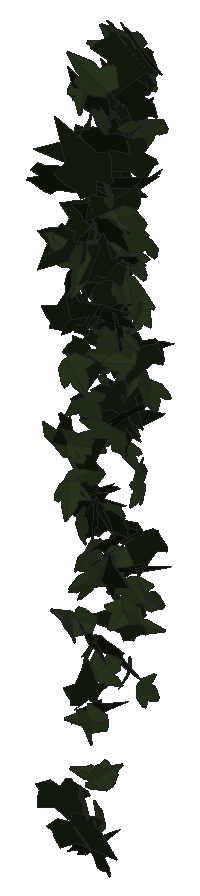
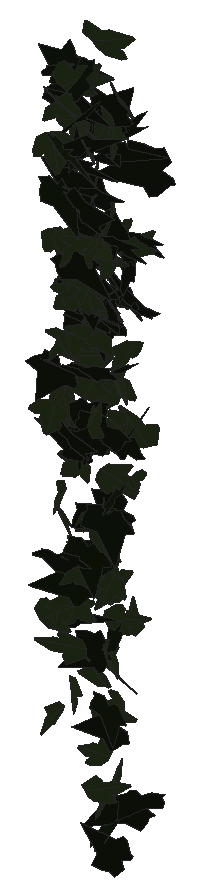
# SketchUp Ruby script. Lengths in inches.
U = 1.inch
M = Sketchup.active_model
def pt(a) = Geom::Point3d.new(a.map { |v| v * U })
def face(e, loops, mat)
  f = e.add_face(loops[0].map { |a| pt(a) })
  loops[1..].each { |l| e.add_face(l.map { |a| pt(a) }).erase! }
  f.material = f.back_material = mat if mat
  f
end
# faces: each face lists its corners as indices into pts; further lists are holes
def faces(e, pts, list, mat = nil) = list.each { |f| face(e, (f[0].is_a?(Array) ? f : [f]).map { |l| l.map { |i| pts[i] } }, mat) }
# xy, xz, yz: faces in a plane at the given z, y or x. An outline is a flat list of corners, or four numbers for a rectangle; further outlines are holes
def ring(l) = l.size == 4 ? [[l[0], l[1]], [l[2], l[1]], [l[2], l[3]], [l[0], l[3]]] : l.each_slice(2).to_a
def flat(e, list, mat, &to3) = list.each { |f| face(e, (f[0].is_a?(Array) ? f : [f]).map { |l| ring(l).map { |u, v| to3.(u, v) } }, mat) }
def xy(e, z, list, mat = nil) = flat(e, list, mat) { |x, y| [x, y, z] }
def xz(e, y, list, mat = nil) = flat(e, list, mat) { |x, z| [x, y, z] }
def yz(e, x, list, mat = nil) = flat(e, list, mat) { |y, z| [x, y, z] }
def lines(e, pts, list) = list.each { |a, b| e.add_line(pt(pts[a]), pt(pts[b])) }
# prism: a flat outline (further loops are holes) pulled along v
def prism(e, loops, v, mat = nil)
  f = face(e, loops, mat); d = Geom::Vector3d.new(v.map { |x| x * U })
  f.pushpull(f.normal.samedirection?(d) ? d.length : -d.length)
end
def box(e, o, s, mat = nil) = prism(e, [[o, [o[0] + s[0], o[1], o[2]], [o[0] + s[0], o[1] + s[1], o[2]], [o[0], o[1] + s[1], o[2]]]], [0, 0, s[2]], mat)
def at(x, y, z, deg = 0) = Geom::Transformation.translation(pt([x, y, z])) * Geom::Transformation.rotation(ORIGIN, Z_AXIS, deg.degrees)
def axes(o, x, y, z) = Geom::Transformation.new([*x, 0, *y, 0, *z, 0, *pt(o).to_a, 1])
def part(name) = M.definitions.add(name)
# library, detail: a bought-in or finely detailed component or shape, given as its bounding box
def library(name, o, s) = part(name).tap { |d| box(d.entities, o, s) }
def detail(e, o, s) = box(e.add_group.entities, o, s)
def put(e, d, t, mat = nil) = e.add_instance(d, t).tap { |i| i.material = mat if mat }
def group(e, t, mat = nil) = e.add_group.tap { |g| g.transformation = t; g.material = mat if mat }.entities
root = M.entities
M.materials.add("1026 AP 7946 SUNNY SIDE UP").color = [254, 231, 186]
M.materials.add("efeu1").color = [18, 25, 13]
M.materials.add("efeu2").color = [43, 57, 29]
c1 = part("ivyleaf_10")
p = [[0,0.5,-0.03],[-0.0625,2.02,-0.43],[-0.19,2.01,-0.46],[-0.54,1.05,-0.29],[-0.52,0.625,-0.18],[-0.83,0.76,-0.28],
  [-1.16,0.64,-0.33],[-1.15,0.33,-0.24],[-0.77,-0.39,0.02],[-0.3,-0.51,0.16],[0.04,-0.48,0.23],[-0.02,2.01,-0.4375],
  [-0.06,2.01,-0.43],[0.04,-0.49,0.23],[0.67,-0.49,0.14],[1.38,0.36,-0.2],[1.375,0.51,-0.24],[0.81,0.65,-0.19],
  [0.62,0.59,-0.15],[0.6,1.09,-0.28],[0.5,1.23,-0.31]]
faces(c1.entities,p,[[0,1,2,3,4,5,6,7,8,9,10],[11,12,0,13,14,15,16,17,18,19,20]],"efeu2")
c2 = part("ivyleaf_9")
p = [[1.54,2.16,1.25],[1.36,2.04,1.19],[-0.21,0.99,0.68],[-0.71,1.11,0.82],[-0.85,0.86,0.67],[-0.8,0.17,0.21],
  [-0.9,-0.01,0.1],[-0.67,-0.16,-0.02],[-0.08,-0.08,-0.05],[-0.03,-0.6,-0.4],[0.65,-0.88,-0.66],[0.83,-0.6,-0.49],
  [1.29,-0.42,-0.43],[1.8125,-0.07,-0.26],[1.21,0.44,0.15]]
faces(c2.entities,p,[[0,1,2,3,4,5,6,7,8,9,10,11,12,13,14]],"efeu1")
put(root,c1,axes([143.42,211.94,263.75],[0.0938,-0.15125,0.23825],[-0.1014,0.22334,0.1683],[-0.42367,-0.08694,0.01247]),"1026 AP 7946 SUNNY SIDE UP")
put(root,c1,axes([143.43,211.76,261.33],[0.13423,-0.24089,0.02865],[0.00299,-0.03026,-0.26333],[0.38153,0.08499,-0.00801]),"1026 AP 7946 SUNNY SIDE UP")
put(root,c2,axes([143.54,211.24,263.9375],[-0.37128,-0.07573,0.00381],[0.00504,-0.02344,-0.25446],[0.11914,-0.23499,0.02262]),"1026 AP 7946 SUNNY SIDE UP")
put(root,c2,axes([143.59,211.95,264.14],[-0.42703,-0.09368,0.03011],[-0.02533,-0.04383,-0.29388],[0.15246,-0.26966,0.0355]),"1026 AP 7946 SUNNY SIDE UP")
put(root,c2,axes([143.54,211.85,258.47],[0.05473,0.28173,-0.03546],[-0.00171,-0.03616,-0.29264],[-0.4466,0.03466,-0.00322]),"1026 AP 7946 SUNNY SIDE UP")
put(root,c1,axes([143.47,212.01,262.93],[0.05377,0.17538,-0.17233],[0.00628,0.16951,0.18382],[0.38213,-0.02746,0.02123]),"1026 AP 7946 SUNNY SIDE UP")
put(root,c2,axes([143.3,211.23,252.57],[-0.07006,-0.19758,-0.17581],[0.07492,0.16291,-0.20754],[0.40246,-0.06472,0.00803]),"1026 AP 7946 SUNNY SIDE UP")
put(root,c1,axes([143.41,211.89,257.2],[-0.08145,-0.1963,-0.19583],[0.11754,0.17474,-0.20708],[0.41201,-0.08865,0.02036]),"1026 AP 7946 SUNNY SIDE UP")
put(root,c1,axes([143.55,211.19,263.64],[0.19022,0.18463,0.11983],[-0.11789,-0.08845,0.22651],[0.32129,-0.14176,0.01217]),"1026 AP 7946 SUNNY SIDE UP")
put(root,c2,axes([143.13,210.93,265.28],[0.36968,0.0612,0.20377],[0.31158,0.01846,-0.24885],[-0.09259,0.30647,-0.02384]),"1026 AP 7946 SUNNY SIDE UP")
put(root,c2,axes([143.57,211.21,263.37],[0.03211,-0.04656,-0.25738],[-0.28074,0.17538,-0.04773],[0.28382,0.17874,-0.01809]),"1026 AP 7946 SUNNY SIDE UP")
put(root,c1,axes([143.43,212.49,264.14],[-0.01526,0.013,0.27735],[0.1577,-0.2498,0.01469],[0.39327,0.10067,0.00487]),"1026 AP 7946 SUNNY SIDE UP")
put(root,c1,axes([143.6,212.22,260.48],[-0.25335,0.18288,-0.06389],[-0.04568,0.05826,0.25088],[0.30073,0.16292,-0.01572]),"1026 AP 7946 SUNNY SIDE UP")
put(root,c1,axes([143.76,211.39,256.09],[-0.06083,-0.04387,-0.23084],[-0.33816,-0.0686,0.05174],[-0.11945,0.21654,-0.02893]),"1026 AP 7946 SUNNY SIDE UP")
put(root,c2,axes([143.83,211.62,265.67],[-0.27226,-0.02774,0.24253],[-0.34908,-0.08377,-0.17875],[0.13135,-0.28011,0.02764]),"1026 AP 7946 SUNNY SIDE UP")
put(root,c2,axes([143.65,211.71,266.58],[0.19878,-0.08871,0.20137],[-0.22642,0.13397,0.15896],[-0.25128,-0.19089,0.01607]),"1026 AP 7946 SUNNY SIDE UP")
put(root,c2,axes([143.45,211.34,259.96],[0.12325,-0.16914,-0.19309],[0.19016,-0.146,0.18794],[-0.34719,-0.14001,0.03439]),"1026 AP 7946 SUNNY SIDE UP")
put(root,c2,axes([143.66,211.25,263.76],[-0.01751,0.15665,0.20459],[-0.01072,0.19764,-0.16056],[-0.39648,-0.01226,-0.00469]),"1026 AP 7946 SUNNY SIDE UP")
put(root,c2,axes([143.51,211.96,263.05],[-0.26418,0.01414,-0.19195],[0.27194,-0.0834,-0.16759],[-0.11161,-0.23668,0.04603]),"1026 AP 7946 SUNNY SIDE UP")
put(root,c1,axes([143.41,211.67,266.95],[0.28547,-0.11304,0.13228],[0.15325,-0.08666,-0.21997],[0.222,0.20519,-0.01825]),"1026 AP 7946 SUNNY SIDE UP")
put(root,c1,axes([143.37,211.08,259.79],[-0.32254,0.01111,0.17998],[0.27502,0.02193,0.21032],[-0.00912,0.26851,-0.02305]),"1026 AP 7946 SUNNY SIDE UP")
put(root,c2,axes([143.78,212.48,266.16],[-0.16257,0.0006,0.24877],[-0.3352,-0.12362,-0.09444],[0.17837,-0.23177,0.04927]),"1026 AP 7946 SUNNY SIDE UP")
put(root,c1,axes([143.6,211.62,266.25],[0.02906,-0.21847,-0.12434],[-0.0006,0.11976,-0.225],[0.39153,0.0164,0.00889]),"1026 AP 7946 SUNNY SIDE UP")
put(root,c1,axes([143.5625,211.16,255.94],[-0.28361,0.1433,0.05702],[0.07891,-0.02439,0.23686],[0.22781,0.18684,-0.01106]),"1026 AP 7946 SUNNY SIDE UP")
put(root,c1,axes([143.81,212.43,263.23],[-0.27014,-0.07664,0.20533],[-0.24592,-0.12981,-0.19065],[0.22955,-0.22926,0.03739]),"1026 AP 7946 SUNNY SIDE UP")
put(root,c2,axes([143.5,211.83,261.4],[-0.09596,-0.24897,0.04401],[-0.00448,-0.04472,-0.26422],[0.39755,-0.0606,0.00765]),"1026 AP 7946 SUNNY SIDE UP")
put(root,c1,axes([143.74,211.58,259.14],[-0.15307,-0.11435,0.20737],[-0.15059,-0.17968,-0.15343],[0.33239,-0.13407,0.02599]),"1026 AP 7946 SUNNY SIDE UP")
put(root,c1,axes([143.53,211.8,264.61],[-0.14488,0.27122,-0.06508],[0.00856,-0.06639,-0.29503],[-0.43835,-0.09094,0.01575]),"1026 AP 7946 SUNNY SIDE UP")
put(root,c2,axes([143.73,212.08,263.15],[0.05998,0.19402,-0.19439],[-0.08197,-0.18286,-0.20443],[-0.41883,0.06357,0.01217]),"1026 AP 7946 SUNNY SIDE UP")
put(root,c2,axes([143.67,211.09,262.37],[-0.38093,0.04621,0.0685],[0.10943,0.01319,0.25283],[0.06442,0.25081,-0.02439]),"1026 AP 7946 SUNNY SIDE UP")
put(root,c2,axes([143.71,211.625,254.43],[-0.00749,0.24032,0.06934],[-0.00029,0.06595,-0.24723],[-0.39184,-0.00464,-0.00115]),"1026 AP 7946 SUNNY SIDE UP")
put(root,c2,axes([143.87,212.22,264.75],[-0.03104,0.04182,0.27883],[-0.25401,0.21705,-0.04546],[-0.34728,-0.16249,0.00833]),"1026 AP 7946 SUNNY SIDE UP")
put(root,c1,axes([143.43,212.43,262.48],[-0.33186,-0.08937,-0.16155],[0.27561,-0.04686,-0.21648],[0.06479,-0.25842,0.09339]),"1026 AP 7946 SUNNY SIDE UP")
put(root,c2,axes([143.83,212.5,263.88],[0.07244,0.04148,-0.25277],[-0.30772,-0.14848,-0.06452],[-0.24228,0.20099,0.00637]),"1026 AP 7946 SUNNY SIDE UP")
put(root,c1,axes([143.7,211.3,258.11],[-0.09191,0.12654,0.2231],[-0.16776,0.18788,-0.14214],[-0.35585,-0.12126,0.00939]),"1026 AP 7946 SUNNY SIDE UP")
put(root,c1,axes([143.59,211.11,258.9],[0.12972,0.23931,-0.07447],[-0.03065,-0.07116,-0.26115],[-0.39251,0.08464,-0.00422]),"1026 AP 7946 SUNNY SIDE UP")
put(root,c1,axes([143.86,212.55,267.54],[-0.24653,-0.08123,-0.2089],[-0.28526,-0.08958,0.18137],[-0.1901,0.23977,-0.00126]),"1026 AP 7946 SUNNY SIDE UP")
put(root,c1,axes([143.77,212.17,261.1],[-0.19965,-0.1653,-0.14258],[-0.15538,-0.09691,0.21352],[-0.30022,0.16008,-0.01569]),"1026 AP 7946 SUNNY SIDE UP")
put(root,c1,axes([143.67,212.36,263.21],[0.39344,-0.12703,-0.02329],[-0.0408,-0.00283,-0.28873],[0.19854,0.25115,-0.01318]),"1026 AP 7946 SUNNY SIDE UP")
put(root,c1,axes([143.65,212.03,264.06],[0.03212,0.15736,-0.19606],[-0.042,-0.18934,-0.16457],[-0.38711,0.0336,0.00159]),"1026 AP 7946 SUNNY SIDE UP")
put(root,c1,axes([143.98,211.76,263.65],[0.08927,0.04365,0.26573],[-0.40542,-0.03382,0.06423],[0.06729,-0.26169,0.03443]),"1026 AP 7946 SUNNY SIDE UP")
put(root,c2,axes([143.56,211.59,254.0625],[0.00469,0.17467,-0.18573],[-0.00864,0.18129,0.18092],[0.39573,0.00189,0.00615]),"1026 AP 7946 SUNNY SIDE UP")
put(root,c1,axes([143.73,211.6,255.54],[0.09859,-0.23893,0.02508],[0.00498,-0.02574,-0.25461],[0.37783,0.06269,-0.00319]),"1026 AP 7946 SUNNY SIDE UP")
put(root,c2,axes([143.8,212.11,263.29],[0.18323,0.24002,-0.09196],[-0.11272,-0.06511,-0.27299],[-0.38734,0.13249,0.03594]),"1026 AP 7946 SUNNY SIDE UP")
put(root,c2,axes([143.6,211.51,255.93],[0.29277,-0.15351,-0.12378],[-0.16446,0.06012,-0.24756],[0.25768,0.21279,-0.01736]),"1026 AP 7946 SUNNY SIDE UP")
put(root,c1,axes([143.65,211.79,266.48],[-0.31533,0.18522,-0.08686],[0.07102,-0.07641,-0.28056],[-0.31272,-0.20412,0.02386]),"1026 AP 7946 SUNNY SIDE UP")
put(root,c1,axes([143.89,211.78,252.72],[0.07757,0.08925,0.22574],[-0.20719,-0.17492,0.10318],[0.3081,-0.1401,0.01255]),"1026 AP 7946 SUNNY SIDE UP")
put(root,c2,axes([143.57,211.46,258.41],[0.23544,0.14667,0.18944],[0.21516,0.12177,-0.21511],[-0.29957,0.20274,-0.00561]),"1026 AP 7946 SUNNY SIDE UP")
put(root,c1,axes([143.7,211.58,256.85],[-0.00607,0.04573,0.30029],[0.09848,-0.28448,0.04521],[0.45297,0.06246,-0.00581]),"1026 AP 7946 SUNNY SIDE UP")
put(root,c1,axes([143.8125,211.77,258.29],[-0.35545,-0.17911,0.02597],[-0.01061,-0.03359,-0.29645],[0.28444,-0.22508,0.0214]),"1026 AP 7946 SUNNY SIDE UP")
put(root,c1,axes([143.75,212.33,266.45],[0.18119,-0.26601,0.0492],[0.01693,-0.049,-0.29878],[0.42506,0.11535,-0.00907]),"1026 AP 7946 SUNNY SIDE UP")
put(root,c2,axes([143.86,211.64,258.3],[0.26615,0.09662,-0.22143],[-0.26739,-0.1341,-0.20033],[-0.25766,0.23896,-0.02083]),"1026 AP 7946 SUNNY SIDE UP")
put(root,c2,axes([143.87,211.65,264.35],[0.35396,0.04472,-0.26931],[-0.40132,-0.0579,-0.23673],[-0.1148,0.34029,-0.00281]),"1026 AP 7946 SUNNY SIDE UP")
put(root,c2,axes([143.54,211.71,258.75],[0.20838,-0.26132,0.0119],[-0.01702,-0.02008,-0.30135],[0.41106,0.13164,-0.01851]),"1026 AP 7946 SUNNY SIDE UP")
put(root,c2,axes([143.99,212.41,260.13],[-0.03891,0.0812,0.23432],[-0.22078,0.18063,-0.08128],[-0.30813,-0.13968,0.02865]),"1026 AP 7946 SUNNY SIDE UP")
put(root,c2,axes([143.88,210.97,262.51],[-0.27177,0.14284,-0.14491],[-0.1447,0.10966,0.23053],[0.28105,0.19458,-0.02143]),"1026 AP 7946 SUNNY SIDE UP")
put(root,c2,axes([143.6875,212.28,261.625],[-0.22978,-0.17369,-0.10989],[0.12682,0.06995,-0.23292],[0.29347,-0.16623,0.01461]),"1026 AP 7946 SUNNY SIDE UP")
put(root,c1,axes([144,212.35,267.44],[0.07148,0.09983,0.26681],[-0.30038,-0.17837,0.10456],[0.3155,-0.19244,0.0391]),"1026 AP 7946 SUNNY SIDE UP")
put(root,c1,axes([143.6875,211.03,261.51],[0.08199,0.2633,0.10856],[0.02108,0.10322,-0.27584],[-0.44458,0.05345,0.00694]),"1026 AP 7946 SUNNY SIDE UP")
put(root,c2,axes([143.85,212.17,262.61],[-0.38483,-0.12176,-0.02761],[0.0603,-0.01893,-0.27955],[0.18628,-0.2454,0.03346]),"1026 AP 7946 SUNNY SIDE UP")
put(root,c2,axes([143.59,211.48,251.3125],[0.20779,0.21359,-0.00679],[-0.01252,0.01409,0.25842],[0.33584,-0.13162,0.01384]),"1026 AP 7946 SUNNY SIDE UP")
put(root,c1,axes([143.62,212.31,264.18],[0.1568,0.19053,0.19197],[0.1287,0.16624,-0.22054],[-0.39756,0.12896,0.00432]),"1026 AP 7946 SUNNY SIDE UP")
put(root,c2,axes([143.52,212.55,267.72],[0.32986,-0.19791,0.04758],[0.03156,-0.04749,-0.29664],[0.3184,0.20974,-0.01989]),"1026 AP 7946 SUNNY SIDE UP")
put(root,c2,axes([143.51,211.97,260.37],[-0.02944,-0.08156,-0.2823],[0.32664,0.18414,-0.07012],[0.30786,-0.20317,0.04741]),"1026 AP 7946 SUNNY SIDE UP")
put(root,c2,axes([143.61,211.28,259.53],[-0.12219,0.07975,0.24342],[0.26726,-0.16353,0.11371],[0.28603,0.18686,-0.00225]),"1026 AP 7946 SUNNY SIDE UP")
put(root,c1,axes([143.93,212.06,261.43],[-0.02579,-0.04315,-0.27257],[-0.21078,-0.22795,0.04557],[-0.3646,0.13483,-0.00706]),"1026 AP 7946 SUNNY SIDE UP")
put(root,c1,axes([144.04,211.41,254.13],[-0.03449,0.00152,0.22443],[-0.25749,-0.14452,-0.01679],[0.22592,-0.16448,0.01512]),"1026 AP 7946 SUNNY SIDE UP")
put(root,c1,axes([144.01,211.84,256.96],[-0.21155,-0.07613,0.16404],[-0.19102,-0.10603,-0.15817],[0.20216,-0.17986,0.02221]),"1026 AP 7946 SUNNY SIDE UP")
put(root,c1,axes([143.99,211.88,261.83],[-0.3936,0.02015,0.11061],[-0.1713,-0.0303,-0.25624],[-0.01013,-0.27064,0.03532]),"1026 AP 7946 SUNNY SIDE UP")
put(root,c2,axes([143.84,211.72,262.41],[0.31974,0.13038,-0.12909],[-0.14681,-0.08708,-0.24848],[-0.24446,0.22283,-0.01962]),"1026 AP 7946 SUNNY SIDE UP")
put(root,c1,axes([144.09,212.35,264.1875],[-0.23988,0.00737,0.19512],[-0.29585,-0.03489,-0.15497],[0.03555,-0.24065,0.02701]),"1026 AP 7946 SUNNY SIDE UP")
put(root,c2,axes([143.99,212.28,266.48],[-0.16537,-0.2226,0.11404],[0.05701,0.10656,0.25397],[-0.38763,0.11064,-0.0113]),"1026 AP 7946 SUNNY SIDE UP")
put(root,c2,axes([143.99,211.1,254.78],[-0.32396,0.11744,-0.05732],[-0.06637,0.03949,0.24417],[0.19374,0.2099,-0.01221]),"1026 AP 7946 SUNNY SIDE UP")
put(root,c2,axes([143.97,211.8,262.46],[0.09672,0.24013,-0.12578],[-0.03841,-0.12115,-0.25601],[-0.42283,0.06594,-0.00551]),"1026 AP 7946 SUNNY SIDE UP")
put(root,c1,axes([143.76,212.52,263.23],[-0.32645,-0.00555,-0.12637],[0.1914,-0.04053,-0.21064],[-0.02501,-0.23769,0.03744]),"1026 AP 7946 SUNNY SIDE UP")
put(root,c2,axes([143.98,211.89,257.67],[0.03547,0.27988,-0.01364],[0.00981,-0.01538,-0.28926],[-0.4406,0.02219,-0.00754]),"1026 AP 7946 SUNNY SIDE UP")
put(root,c1,axes([143.82,212.61,262.36],[0.39973,0.01878,0.01802],[0.03004,-0.02372,-0.26148],[-0.02678,0.2537,-0.02428]),"1026 AP 7946 SUNNY SIDE UP")
put(root,c2,axes([143.71,211.1,262.48],[-0.05399,0.11155,0.23595],[0.16014,-0.20513,0.11779],[0.36621,0.10615,-0.01672]),"1026 AP 7946 SUNNY SIDE UP")
put(root,c1,axes([143.875,211.15,263.78],[0.07062,0.28095,-0.22232],[-0.05567,-0.2145,-0.29436],[-0.55579,0.05719,0.00124]),"1026 AP 7946 SUNNY SIDE UP")
put(root,c2,axes([144.14,212.53,266.21],[-0.31236,0.20159,-0.01267],[-0.00718,-0.02333,-0.291],[-0.3176,-0.19773,0.01904]),"1026 AP 7946 SUNNY SIDE UP")
put(root,c2,axes([143.77,212.35,265.95],[0.22014,-0.18027,-0.18551],[0.20839,-0.12261,0.23321],[-0.34086,-0.19138,0.02276]),"1026 AP 7946 SUNNY SIDE UP")
put(root,c1,axes([143.97,211.61,257.32],[-0.09311,-0.26492,0.02743],[-0.00064,-0.02872,-0.27976],[0.4189,-0.05893,0.00567]),"1026 AP 7946 SUNNY SIDE UP")
put(root,c1,axes([143.88,211.22,260.78],[-0.18676,-0.20764,-0.14006],[0.12722,0.10871,-0.24537],[0.36787,-0.14301,0.01375]),"1026 AP 7946 SUNNY SIDE UP")
put(root,c2,axes([144.05,211.55,266.18],[0.13899,0.14439,-0.20011],[-0.13637,-0.17509,-0.17503],[-0.3564,0.1233,-0.01106]),"1026 AP 7946 SUNNY SIDE UP")
put(root,c1,axes([143.82,211.05,259.92],[0.05635,0.08254,0.25103],[0.06726,0.24021,-0.08908],[-0.3982,0.05226,0.02048]),"1026 AP 7946 SUNNY SIDE UP")
put(root,c2,axes([144.04,212.01,265],[-0.42067,-0.14251,-0.00515],[0.02927,-0.02609,-0.31071],[0.22227,-0.26629,0.03118]),"1026 AP 7946 SUNNY SIDE UP")
put(root,c1,axes([143.83,211.18,254.26],[-0.18572,0.13583,-0.14073],[0.11545,-0.11737,-0.18527],[-0.28097,-0.138,0.01689]),"1026 AP 7946 SUNNY SIDE UP")
put(root,c1,axes([143.71,212.125,261.84],[-0.18376,0.00052,-0.21275],[0.31777,-0.04858,-0.11823],[-0.06688,-0.23227,0.02283]),"1026 AP 7946 SUNNY SIDE UP")
put(root,c1,axes([143.88,212.46,263.4375],[-0.11016,0.13194,0.20937],[0.13971,-0.182,0.15277],[0.3534,0.11308,0.00487]),"1026 AP 7946 SUNNY SIDE UP")
put(root,c1,axes([144.11,211.59,260.08],[-0.3593,-0.06153,0.11916],[-0.16522,-0.05401,-0.24302],[0.12387,-0.25051,0.0215]),"1026 AP 7946 SUNNY SIDE UP")
put(root,c1,axes([143.95,212.05,262.77],[-0.26222,0.21071,-0.06474],[-0.00055,-0.08058,-0.27268],[-0.34629,-0.15943,0.04946]),"1026 AP 7946 SUNNY SIDE UP")
put(root,c2,axes([144.2,211.0625,265.57],[-0.32194,-0.28548,0.11115],[0.07266,0.1014,0.36189],[-0.47526,0.20889,-0.01997]),"1026 AP 7946 SUNNY SIDE UP")
put(root,c1,axes([143.79,212.45,263.47],[-0.27623,0.09819,-0.19351],[0.23942,-0.11229,-0.20721],[-0.23296,-0.23183,0.0165]),"1026 AP 7946 SUNNY SIDE UP")
put(root,c2,axes([143.75,211,252.1],[-0.02336,-0.08073,-0.27304],[0.16644,0.24313,-0.08112],[0.40185,-0.10539,0.01773]),"1026 AP 7946 SUNNY SIDE UP")
put(root,c2,axes([144.27,212.26,266.79],[-0.12963,0.19142,0.20221],[-0.20045,0.15345,-0.20959],[-0.3803,-0.14613,0.04154]),"1026 AP 7946 SUNNY SIDE UP")
put(root,c1,axes([144.05,212.59,267.03],[0.17889,0.17595,-0.19327],[-0.16595,-0.15633,-0.21675],[-0.37007,0.15516,0.00377]),"1026 AP 7946 SUNNY SIDE UP")
put(root,c1,axes([144,211.76,264.86],[-0.22158,0.23594,0.08157],[0.07955,-0.06036,0.28249],[0.38248,0.14924,-0.0115]),"1026 AP 7946 SUNNY SIDE UP")
put(root,c1,axes([144.02,212.05,257.29],[0.17964,0.20957,-0.13125],[-0.10594,-0.10969,-0.24646],[-0.37182,0.1325,0.00681]),"1026 AP 7946 SUNNY SIDE UP")
put(root,c2,axes([143.7,212.23,259.91],[0.01632,0.0279,0.27893],[0.40666,-0.085,-0.00169],[0.13267,0.25711,-0.02914]),"1026 AP 7946 SUNNY SIDE UP")
put(root,c1,axes([144.06,211,252.48],[-0.21165,0.19299,-0.00854],[0.0049,0.01361,0.24225],[0.30378,0.13424,-0.00986]),"1026 AP 7946 SUNNY SIDE UP")
put(root,c2,axes([143.9,212,260.68],[-0.01434,-0.17335,-0.20894],[0.02475,0.20125,-0.17762],[0.41762,-0.01788,0.00335]),"1026 AP 7946 SUNNY SIDE UP")
put(root,c1,axes([143.84,211.72,254.98],[0.32462,-0.10197,-0.1312],[0.19544,-0.0333,0.23593],[-0.16507,-0.23997,0.02133]),"1026 AP 7946 SUNNY SIDE UP")
put(root,c2,axes([143.92,211.48,258.48],[-0.04853,0.00665,-0.25544],[0.31929,-0.14289,-0.03082],[-0.22411,-0.20503,0.01141]),"1026 AP 7946 SUNNY SIDE UP")
put(root,c1,axes([144.21,212.375,261.01],[-0.28563,0.12305,0.1463],[-0.21407,0.04857,-0.22357],[-0.20245,-0.22496,0.02999]),"1026 AP 7946 SUNNY SIDE UP")
put(root,c2,axes([143.95,211.47,257.37],[-0.04198,0.23045,-0.0834],[-0.01061,0.08203,0.23946],[0.3846,0.02742,-0.0025]),"1026 AP 7946 SUNNY SIDE UP")
put(root,c1,axes([144.11,211.38,252.07],[-0.10014,0.19887,-0.00399],[0.00432,0.00613,0.21511],[0.31277,0.06359,-0.00425]),"1026 AP 7946 SUNNY SIDE UP")
put(root,c2,axes([144.09,212.3125,267.61],[-0.33768,-0.21391,-0.03399],[0.04998,0.01307,-0.31189],[0.33635,-0.2167,0.01222]),"1026 AP 7946 SUNNY SIDE UP")
put(root,c2,axes([143.85,211.7,255.5625],[0.39032,-0.0622,0.03261],[0.03927,-0.03143,-0.26264],[0.10275,0.24831,-0.02351]),"1026 AP 7946 SUNNY SIDE UP")
put(root,c2,axes([144.08,212.03,261.8],[-0.07445,0.12611,0.24351],[-0.13416,-0.23394,0.10994],[0.39829,-0.05523,0.08255]),"1026 AP 7946 SUNNY SIDE UP")
put(root,c2,axes([143.91,212.18,259.66],[0.01881,0.00553,0.26427],[0.06912,-0.25302,0.00202],[0.39744,0.04374,-0.01286]),"1026 AP 7946 SUNNY SIDE UP")
put(root,c2,axes([144.17,211.35,251.4],[0.07642,-0.25075,0.04768],[0.00069,0.04864,0.26323],[-0.40135,-0.04766,0.00953]),"1026 AP 7946 SUNNY SIDE UP")
put(root,c2,axes([144.35,212.21,265.64],[-0.43762,-0.04052,0.10071],[-0.13981,-0.06077,-0.28642],[0.09085,-0.28874,0.04435]),"1026 AP 7946 SUNNY SIDE UP")
put(root,c1,axes([144.34,211.07,267.55],[0.29087,0.06218,0.23649],[-0.35914,-0.03303,0.19894],[0.10232,-0.29268,0.02598]),"1026 AP 7946 SUNNY SIDE UP")
put(root,c2,axes([144.47,212.09,266.91],[-0.12006,0.00558,-0.29719],[-0.41293,-0.12505,0.06838],[-0.18809,0.27098,0.0396]),"1026 AP 7946 SUNNY SIDE UP")
put(root,c1,axes([144.17,212.08,254.9375],[0.05327,-0.19253,-0.15102],[-0.04483,0.14271,-0.20053],[0.3768,0.0442,-0.00251]),"1026 AP 7946 SUNNY SIDE UP")
put(root,c1,axes([144.11,212.58,262.12],[0.0335,0.14922,-0.1926],[-0.06588,-0.18333,-0.15603],[-0.37137,0.04598,0.01031]),"1026 AP 7946 SUNNY SIDE UP")
put(root,c1,axes([144.19,212.125,261.26],[-0.05746,0.09839,0.25187],[-0.03499,-0.24655,0.09757],[0.4121,-0.00722,0.0434]),"1026 AP 7946 SUNNY SIDE UP")
put(root,c1,axes([144.02,212.11,259.53],[-0.29838,0.0552,-0.11437],[0.15415,-0.05838,-0.2023],[-0.12006,-0.21212,0.0245]),"1026 AP 7946 SUNNY SIDE UP")
put(root,c2,axes([144.27,211.08,263.63],[-0.33302,0.15103,-0.09667],[-0.0993,0.07394,0.26744],[0.26212,0.2199,-0.02149]),"1026 AP 7946 SUNNY SIDE UP")
put(root,c1,axes([144.08,212.22,256.63],[-0.29733,-0.13624,-0.11146],[0.17208,0.02964,-0.237],[0.2117,-0.21545,0.0361]),"1026 AP 7946 SUNNY SIDE UP")
put(root,c1,axes([144.14,212.35,261.0625],[0.04161,0.20136,-0.15638],[-0.05124,-0.14978,-0.20984],[-0.39428,0.04072,0.01077]),"1026 AP 7946 SUNNY SIDE UP")
put(root,c2,axes([144.24,211.57,263.625],[-0.20355,-0.16362,0.16172],[-0.13679,-0.13225,-0.21541],[0.33034,-0.15558,0.01046]),"1026 AP 7946 SUNNY SIDE UP")
put(root,c1,axes([144.28,212.25,258.87],[-0.02647,0.03845,0.25329],[-0.1815,0.21686,-0.04185],[-0.34627,-0.11661,0.00257]),"1026 AP 7946 SUNNY SIDE UP")
put(root,c2,axes([144.3125,211.91,260.4],[-0.05799,0.23891,-0.09758],[0.02906,-0.09435,-0.24957],[-0.40386,-0.0411,-0.00394]),"1026 AP 7946 SUNNY SIDE UP")
put(root,c2,axes([143.91,211.91,264.9],[0.34441,0.16757,-0.07192],[0.0639,0.06288,0.28335],[0.27879,-0.22142,0.0239]),"1026 AP 7946 SUNNY SIDE UP")
put(root,c1,axes([144.22,212.37,258.58],[0.21817,-0.16539,-0.02377],[-0.03293,0.0113,-0.22215],[0.2603,0.14005,-0.00818]),"1026 AP 7946 SUNNY SIDE UP")
put(root,c2,axes([144.46,211.93,256.13],[-0.24455,-0.03084,0.20353],[-0.28867,-0.07774,-0.16169],[0.12531,-0.23926,0.02473]),"1026 AP 7946 SUNNY SIDE UP")
put(root,c1,axes([144.09,212.3,266.69],[-0.2576,0.13543,-0.19688],[0.14427,-0.17845,-0.2115],[-0.33994,-0.17836,0.05943]),"1026 AP 7946 SUNNY SIDE UP")
put(root,c2,axes([144.22,212.41,261.55],[-0.33068,-0.14259,-0.08202],[0.14785,-0.00115,-0.25637],[0.20919,-0.22458,0.05155]),"1026 AP 7946 SUNNY SIDE UP")
put(root,c2,axes([144.4,212.19,265.05],[-0.0764,0.28975,-0.03912],[0.00061,-0.04009,-0.30283],[-0.45984,-0.04819,0.00609]),"1026 AP 7946 SUNNY SIDE UP")
put(root,c1,axes([144.5,211.79,256.375],[-0.07747,0.01146,0.22113],[-0.33733,-0.01541,-0.04999],[0.01963,-0.21963,0.01375]),"1026 AP 7946 SUNNY SIDE UP")
put(root,c2,axes([144.0625,212,256.97],[0.26861,0.04486,0.2013],[0.23051,0.14671,-0.16609],[-0.21447,0.21387,0.07361]),"1026 AP 7946 SUNNY SIDE UP")
put(root,c1,axes([144.19,211.2,253.1],[-0.04608,-0.11065,0.191],[0.05732,0.18252,0.11883],[-0.33549,0.04639,-0.00593]),"1026 AP 7946 SUNNY SIDE UP")
put(root,c1,axes([144.34,212.43,266.11],[-0.26889,-0.23606,0.02087],[0.00074,-0.02698,-0.29999],[0.37273,-0.17024,0.01566]),"1026 AP 7946 SUNNY SIDE UP")
put(root,c1,axes([143.98,212.25,255.82],[-0.01747,-0.02675,-0.25911],[0.39459,0.02914,-0.01445],[0.04787,-0.24992,0.02455]),"1026 AP 7946 SUNNY SIDE UP")
put(root,c2,axes([144.22,212.4,261.53],[0.24252,0.1872,0.03272],[0.04772,0.0147,-0.24938],[-0.29444,0.15657,-0.01347]),"1026 AP 7946 SUNNY SIDE UP")
put(root,c1,axes([144.28,212.51,260.6875],[-0.39836,-0.00722,-0.03277],[0.05114,-0.04108,-0.25779],[0.00307,-0.252,0.04145]),"1026 AP 7946 SUNNY SIDE UP")
put(root,c1,axes([144.51,212.36,256.32],[-0.25522,0.01136,-0.1742],[-0.26348,0.02492,0.1675],[0.04061,0.23311,-0.00804]),"1026 AP 7946 SUNNY SIDE UP")
put(root,c2,axes([143.99,211.66,257.16],[0.18578,-0.1369,-0.20761],[0.36718,0.00226,0.14001],[-0.10563,-0.23292,0.12155]),"1026 AP 7946 SUNNY SIDE UP")
put(root,c1,axes([144.33,211.84,256.38],[0.23373,0.1251,-0.12566],[-0.132,-0.09037,-0.20024],[-0.24184,0.17024,-0.01214]),"1026 AP 7946 SUNNY SIDE UP")
put(root,c1,axes([144.52,212.12,263.96],[-0.3172,0.05349,0.1754],[-0.26962,0.01149,-0.21333],[-0.07614,-0.26353,0.02469]),"1026 AP 7946 SUNNY SIDE UP")
put(root,c1,axes([144.29,212.36,254.47],[-0.01618,0.15497,0.1902],[-0.04768,0.18161,-0.15848],[-0.37494,-0.02978,0.01194]),"1026 AP 7946 SUNNY SIDE UP")
put(root,c2,axes([144.02,212.44,267.68],[0.14694,-0.14982,0.22947],[0.14789,-0.20358,-0.18222],[0.39652,0.13145,-0.01707]),"1026 AP 7946 SUNNY SIDE UP")
put(root,c2,axes([144.26,212.39,257.66],[-0.27076,-0.1544,-0.10709],[0.13906,0.05538,-0.23735],[0.25666,-0.19289,0.01563]),"1026 AP 7946 SUNNY SIDE UP")
put(root,c1,axes([144.13,212.11,262.89],[0.33954,-0.05731,0.13005],[0.19073,-0.03627,-0.23034],[0.10651,0.24765,-0.00209]),"1026 AP 7946 SUNNY SIDE UP")
